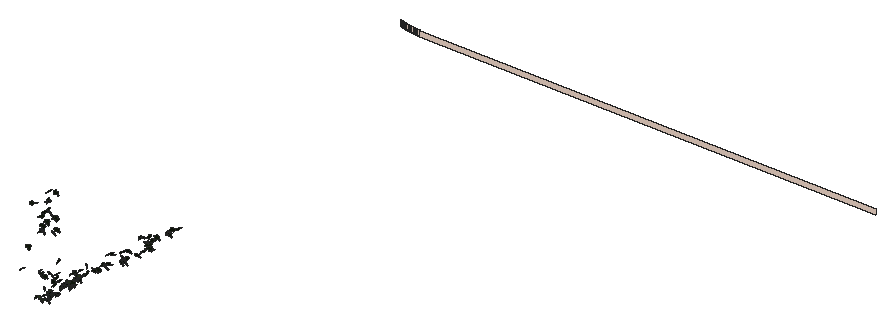
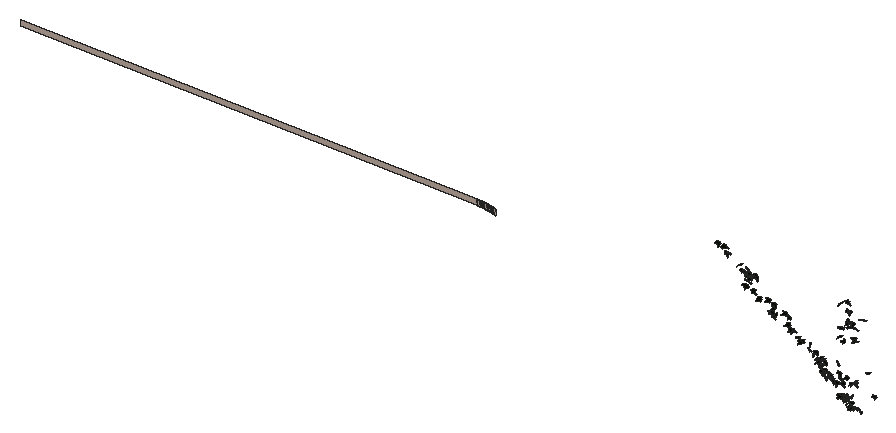
# SketchUp Ruby script. Lengths in inches.
U = 1.inch
M = Sketchup.active_model
def pt(a) = Geom::Point3d.new(a.map { |v| v * U })
def face(e, loops, mat)
  f = e.add_face(loops[0].map { |a| pt(a) })
  loops[1..].each { |l| e.add_face(l.map { |a| pt(a) }).erase! }
  f.material = f.back_material = mat if mat
  f
end
# faces: each face lists its corners as indices into pts; further lists are holes
def faces(e, pts, list, mat = nil) = list.each { |f| face(e, (f[0].is_a?(Array) ? f : [f]).map { |l| l.map { |i| pts[i] } }, mat) }
# xy, xz, yz: faces in a plane at the given z, y or x. An outline is a flat list of corners, or four numbers for a rectangle; further outlines are holes
def ring(l) = l.size == 4 ? [[l[0], l[1]], [l[2], l[1]], [l[2], l[3]], [l[0], l[3]]] : l.each_slice(2).to_a
def flat(e, list, mat, &to3) = list.each { |f| face(e, (f[0].is_a?(Array) ? f : [f]).map { |l| ring(l).map { |u, v| to3.(u, v) } }, mat) }
def xy(e, z, list, mat = nil) = flat(e, list, mat) { |x, y| [x, y, z] }
def xz(e, y, list, mat = nil) = flat(e, list, mat) { |x, z| [x, y, z] }
def yz(e, x, list, mat = nil) = flat(e, list, mat) { |y, z| [x, y, z] }
def lines(e, pts, list) = list.each { |a, b| e.add_line(pt(pts[a]), pt(pts[b])) }
# prism: a flat outline (further loops are holes) pulled along v
def prism(e, loops, v, mat = nil)
  f = face(e, loops, mat); d = Geom::Vector3d.new(v.map { |x| x * U })
  f.pushpull(f.normal.samedirection?(d) ? d.length : -d.length)
end
def box(e, o, s, mat = nil) = prism(e, [[o, [o[0] + s[0], o[1], o[2]], [o[0] + s[0], o[1] + s[1], o[2]], [o[0], o[1] + s[1], o[2]]]], [0, 0, s[2]], mat)
def at(x, y, z, deg = 0) = Geom::Transformation.translation(pt([x, y, z])) * Geom::Transformation.rotation(ORIGIN, Z_AXIS, deg.degrees)
def axes(o, x, y, z) = Geom::Transformation.new([*x, 0, *y, 0, *z, 0, *pt(o).to_a, 1])
def part(name) = M.definitions.add(name)
# library, detail: a bought-in or finely detailed component or shape, given as its bounding box
def library(name, o, s) = part(name).tap { |d| box(d.entities, o, s) }
def detail(e, o, s) = box(e.add_group.entities, o, s)
def put(e, d, t, mat = nil) = e.add_instance(d, t).tap { |i| i.material = mat if mat }
def group(e, t, mat = nil) = e.add_group.tap { |g| g.transformation = t; g.material = mat if mat }.entities
root = M.entities
M.materials.add("1026 AP 7946 SUNNY SIDE UP").color = [254, 231, 186]
M.materials.add("1937 AP K247 Camellia Bud-N").color = [246, 221, 207]
M.materials.add("efeu1").color = [18, 25, 13]
M.materials.add("efeu2").color = [43, 57, 29]
c1 = part("ivyleaf_10")
p = [[0,0.5,-0.03],[-0.0625,2.02,-0.43],[-0.19,2.01,-0.46],[-0.54,1.05,-0.29],[-0.52,0.625,-0.18],[-0.83,0.76,-0.28],
  [-1.16,0.64,-0.33],[-1.15,0.33,-0.24],[-0.77,-0.39,0.02],[-0.3,-0.51,0.16],[0.04,-0.48,0.23],[-0.02,2.01,-0.4375],
  [-0.06,2.01,-0.43],[0.04,-0.49,0.23],[0.67,-0.49,0.14],[1.38,0.36,-0.2],[1.375,0.51,-0.24],[0.81,0.65,-0.19],
  [0.62,0.59,-0.15],[0.6,1.09,-0.28],[0.5,1.23,-0.31]]
faces(c1.entities,p,[[0,1,2,3,4,5,6,7,8,9,10],[11,12,0,13,14,15,16,17,18,19,20]],"efeu2")
c2 = part("ivyleaf_9")
p = [[1.54,2.16,1.25],[1.36,2.04,1.19],[-0.21,0.99,0.68],[-0.71,1.11,0.82],[-0.85,0.86,0.67],[-0.8,0.17,0.21],
  [-0.9,-0.01,0.1],[-0.67,-0.16,-0.02],[-0.08,-0.08,-0.05],[-0.03,-0.6,-0.4],[0.65,-0.88,-0.66],[0.83,-0.6,-0.49],
  [1.29,-0.42,-0.43],[1.8125,-0.07,-0.26],[1.21,0.44,0.15]]
faces(c2.entities,p,[[0,1,2,3,4,5,6,7,8,9,10,11,12,13,14]],"efeu1")
xz(root,299,[[224.73,370,225,372],[225,370,396,372]],"1937 AP K247 Camellia Bud-N")
xz(root,299.01,[[224.2,370,224.47,372]],"1937 AP K247 Camellia Bud-N")
p = [[223.41,299.05,372],[223.15,299.0625,372],[223.15,299.0625,370],[223.41,299.05,370],[223.68,299.03,372],[223.68,299.03,370],
  [223.94,299.02,372],[223.94,299.02,370],[224.2,299.01,372],[224.2,299.01,370],[224.73,299,372],[224.47,299.01,372],
  [224.47,299.01,370],[224.73,299,370],[222.35,299.13,372],[222.09,299.16,372],[222.09,299.16,370],[222.35,299.13,370],
  [222.62,299.11,372],[222.62,299.11,370],[222.88,299.08,372],[222.88,299.08,370],[221.5625,299.22,372],[221.3,299.25,372],
  [221.3,299.25,370],[221.5625,299.22,370],[221.83,299.1875,372],[221.83,299.1875,370],[220.78,299.33,372],[220.51,299.375,372],
  [220.51,299.375,370],[220.78,299.33,370],[221.04,299.29,372],[221.04,299.29,370],[220.25,299.42,372],[219.99,299.47,372],
  [219.99,299.47,370],[220.25,299.42,370],[219.73,299.52,372],[219.47,299.57,372],[219.47,299.57,370],[219.73,299.52,370],
  [219.21,299.63,372],[218.96,299.69,372],[218.96,299.69,370],[219.21,299.63,370],[218.7,299.75,372],[218.44,299.81,372],
  [218.44,299.81,370],[218.7,299.75,370],[218.18,299.875,372],[218.18,299.875,370],[217.93,299.94,372],[217.67,300.01,372],
  [217.67,300.01,370],[217.93,299.94,370],[217.42,300.09,372],[217.42,300.09,370],[217.16,300.16,372],[217.16,300.16,370],
  [216.91,300.24,372],[216.66,300.32,372],[216.66,300.32,370],[216.91,300.24,370]]
faces(root,p,[[0,1,2,3],[4,0,3,5],[6,4,5,7],[8,6,7,9],[10,11,12,13],[14,15,16,17],[18,14,17,19],[20,18,19,21],
  [1,20,21,2],[22,23,24,25],[26,22,25,27],[15,26,27,16],[28,29,30,31],[32,28,31,33],[23,32,33,24],[34,35,36,37],
  [29,34,37,30],[38,39,40,41],[35,38,41,36],[42,43,44,45],[39,42,45,40],[46,47,48,49],[43,46,49,44],[47,50,51,48],
  [52,53,54,55],[50,52,55,51],[53,56,57,54],[56,58,59,57],[60,61,62,63],[58,60,63,59]],"1937 AP K247 Camellia Bud-N")
put(root,c1,axes([149.72,216,291.52],[-0.17011,-0.34982,0.04616],[0.18059,-0.08117,-0.35208],[0.52475,-0.08547,0.13613]),"1026 AP 7946 SUNNY SIDE UP")
put(root,c1,axes([149.96,215.9375,291.71],[-0.41211,-0.26062,-0.0123],[0.05123,-0.01799,-0.3791],[0.40692,-0.26168,0.03527]),"1026 AP 7946 SUNNY SIDE UP")
put(root,c2,axes([151.71,216.18,294.14],[0.05702,-0.34851,0.10563],[0.03455,-0.10275,-0.3614],[0.57107,0.04101,0.01132]),"1026 AP 7946 SUNNY SIDE UP")
put(root,c2,axes([152.55,216.18,293.81],[-0.00015,-0.37303,0.06039],[-0.00756,-0.06073,-0.38462],[0.59423,-0.00087,-0.00488]),"1026 AP 7946 SUNNY SIDE UP")
put(root,c2,axes([154.37,216,298.25],[-0.44324,0.24159,-0.06762],[0.04755,-0.06733,-0.38152],[-0.39134,-0.28181,0.03024]),"1026 AP 7946 SUNNY SIDE UP")
put(root,c1,axes([151.59,216.05,294.53],[0.13663,0.35643,-0.09871],[-0.04004,-0.09449,-0.37849],[-0.5798,0.09052,0.00288]),"1026 AP 7946 SUNNY SIDE UP")
put(root,c2,axes([149.6,216.22,314.85],[-0.67915,0.0452,-0.05361],[0.05432,-0.14548,-0.42433],[-0.09414,-0.41003,0.14191]),"1026 AP 7946 SUNNY SIDE UP")
put(root,c1,axes([148.62,216.08,292.08],[0.52629,-0.11382,-0.05801],[-0.09588,-0.0069,-0.36327],[0.17463,0.33923,-0.02464]),"1026 AP 7946 SUNNY SIDE UP")
put(root,c1,axes([151.9375,215.91,294.43],[0.09275,-0.28891,-0.24916],[-0.05487,0.2379,-0.30219],[0.58825,0.06774,0.0111]),"1026 AP 7946 SUNNY SIDE UP")
put(root,c2,axes([152.52,216.21,294.85],[-0.25319,0.21542,-0.25808],[0.11291,-0.25055,-0.26966],[-0.5086,-0.16286,0.06861]),"1026 AP 7946 SUNNY SIDE UP")
put(root,c2,axes([149.81,216.04,299.81],[0.26931,-0.27079,-0.2448],[-0.10884,0.23177,-0.32424],[0.55431,0.17707,0.05527]),"1026 AP 7946 SUNNY SIDE UP")
put(root,c1,axes([148.83,216.29,301.01],[-0.07493,-0.34442,0.19327],[-0.0523,-0.18674,-0.35923],[0.61597,-0.05775,-0.00699]),"1026 AP 7946 SUNNY SIDE UP")
put(root,c1,axes([150.3125,216,295.59],[-0.24963,0.31574,0.11789],[-0.09076,0.09703,-0.36343],[-0.51925,-0.16875,0.00685]),"1026 AP 7946 SUNNY SIDE UP")
put(root,c2,axes([151.2,216.28,318.45],[-0.18343,-0.39792,-0.18257],[0.18595,0.14527,-0.42074],[0.65772,-0.15205,0.06803]),"1026 AP 7946 SUNNY SIDE UP")
put(root,c2,axes([150.63,215.99,299.73],[0.13417,-0.17103,-0.36413],[-0.08066,0.35277,-0.18706],[0.61075,0.08416,0.05529]),"1026 AP 7946 SUNNY SIDE UP")
put(root,c2,axes([149.15,216.26,314.56],[0.47126,-0.31653,0.00167],[-0.0294,-0.0224,-0.44821],[0.49688,0.29889,-0.0281]),"1026 AP 7946 SUNNY SIDE UP")
put(root,c2,axes([158.375,216.1,299.91],[0.52416,0.13091,-0.17564],[-0.21898,-0.10988,-0.36649],[-0.25868,0.35829,-0.04565]),"1026 AP 7946 SUNNY SIDE UP")
put(root,c2,axes([157.85,216.39,299.3],[-0.56526,-0.10682,-0.08152],[0.13503,-0.01473,-0.38447],[0.15882,-0.36767,0.03675]),"1026 AP 7946 SUNNY SIDE UP")
put(root,c2,axes([151.17,216.38,291.91],[0.30277,-0.30922,0.07791],[0.04857,-0.07187,-0.3755],[0.49885,0.19467,-0.01073]),"1026 AP 7946 SUNNY SIDE UP")
put(root,c2,axes([160.84,216.45,301.19],[-0.56238,-0.15305,0.00027],[0.01955,-0.0319,-0.39941],[0.23987,-0.35623,0.03317]),"1026 AP 7946 SUNNY SIDE UP")
put(root,c2,axes([147.28,216,291.45],[0.05899,0.22927,0.27643],[-0.09594,0.26871,-0.22728],[-0.54503,-0.02249,0.06993]),"1026 AP 7946 SUNNY SIDE UP")
put(root,c2,axes([145.36,216.04,322.64],[0.65967,-0.15991,-0.13381],[0.20046,0.43261,-0.12282],[0.25332,0.07408,0.44565]),"1026 AP 7946 SUNNY SIDE UP")
put(root,c2,axes([149.45,216.11,300.07],[-0.27677,0.30741,0.18647],[-0.18521,0.13839,-0.36283],[-0.52802,-0.20968,0.02953]),"1026 AP 7946 SUNNY SIDE UP")
put(root,c2,axes([150.54,216.14,293.44],[0.12426,0.34712,-0.07049],[-0.04558,-0.06555,-0.36687],[-0.55505,0.08309,0.01435]),"1026 AP 7946 SUNNY SIDE UP")
put(root,c2,axes([161.58,216.59,304.66],[-0.02519,-0.07286,-0.40886],[0.02922,-0.39649,0.07197],[-0.63316,-0.0154,0.01959]),"1026 AP 7946 SUNNY SIDE UP")
put(root,c2,axes([156.92,216.22,298.43],[0.48185,0.18604,-0.1307],[-0.14582,-0.09293,-0.36861],[-0.32369,0.3188,-0.02851]),"1026 AP 7946 SUNNY SIDE UP")
put(root,c1,axes([155.96,216.34,297.66],[-0.24146,0.33983,-0.06349],[0.01896,-0.06424,-0.38423],[-0.54329,-0.15328,0.01481]),"1026 AP 7946 SUNNY SIDE UP")
put(root,c2,axes([151.83,216.39,301.24],[0.5563,-0.17456,0.11322],[0.12394,-0.08933,-0.40447],[0.30064,0.35984,-0.04275]),"1026 AP 7946 SUNNY SIDE UP")
put(root,c2,axes([149.31,216.39,314.9],[0.44466,-0.30642,-0.13757],[-0.16022,0.08517,-0.42873],[0.49942,0.30015,-0.01506]),"1026 AP 7946 SUNNY SIDE UP")
put(root,c2,axes([162.43,216.65,303.75],[-0.59992,-0.09624,-0.03499],[0.09509,-0.10968,-0.38646],[0.12892,-0.36695,0.1222]),"1026 AP 7946 SUNNY SIDE UP")
put(root,c2,axes([170.35,216.75,308.71],[-0.35447,-0.35818,0.08055],[0.04249,-0.11008,-0.42876],[0.57559,-0.21246,0.08126]),"1026 AP 7946 SUNNY SIDE UP")
put(root,c1,axes([152.22,216.37,295.1],[-0.24706,-0.12632,0.31631],[0.34102,0.21919,0.20803],[-0.39666,0.26713,-0.01816]),"1026 AP 7946 SUNNY SIDE UP")
put(root,c2,axes([160.28,216.38,303.7],[-0.17467,0.37956,0.00047],[-0.00785,-0.00323,-0.4074],[-0.59678,-0.11105,0.00522]),"1026 AP 7946 SUNNY SIDE UP")
put(root,c2,axes([154.8,216.32,300.44],[-0.25114,0.4049,0.12691],[-0.1082,0.10259,-0.44704],[-0.65557,-0.17204,0.02516]),"1026 AP 7946 SUNNY SIDE UP")
put(root,c1,axes([157.77,216.48,299.5],[-0.06316,0.38089,-0.00176],[-0.00654,-0.00434,-0.39456],[-0.59891,-0.04012,0.0045]),"1026 AP 7946 SUNNY SIDE UP")
put(root,c2,axes([153.32,216.375,298.76],[0.22721,0.04433,0.39953],[0.61087,0.02102,-0.15157],[-0.05547,0.41309,-0.03271]),"1026 AP 7946 SUNNY SIDE UP")
put(root,c1,axes([161.27,216.51,304.64],[-0.21026,0.37622,-0.03857],[0.00182,-0.04157,-0.41137],[-0.59483,-0.13311,0.01238]),"1026 AP 7946 SUNNY SIDE UP")
put(root,c1,axes([163.14,216.64,303.96],[0.2893,0.30713,-0.17555],[-0.11001,-0.15847,-0.36923],[-0.54258,0.19589,-0.01874]),"1026 AP 7946 SUNNY SIDE UP")
put(root,c2,axes([155.01,216.33,301.98],[-0.03033,0.44677,0.03323],[-0.00488,0.02961,-0.46052],[-0.70405,-0.01945,0.00176]),"1026 AP 7946 SUNNY SIDE UP")
put(root,c1,axes([158.74,216.58,300.76],[-0.60532,-0.02173,-0.0108],[0.02271,-0.07568,-0.3898],[0.03029,-0.3776,0.07644]),"1026 AP 7946 SUNNY SIDE UP")
put(root,c1,axes([151.99,216.37,294.98],[-0.01393,-0.22348,-0.30159],[0.08359,0.28772,-0.22723],[0.57146,-0.04753,0.02589]),"1026 AP 7946 SUNNY SIDE UP")
put(root,c1,axes([164.32,216.89,304.61],[-0.04953,0.03206,-0.40968],[-0.01707,-0.39902,-0.03457],[-0.62739,0.00833,0.03328]),"1026 AP 7946 SUNNY SIDE UP")
put(root,c2,axes([168.9375,216.61,307.51],[0.30285,-0.06673,0.38541],[-0.49335,0.20946,0.20591],[-0.33817,-0.36533,0.04475]),"1026 AP 7946 SUNNY SIDE UP")
put(root,c2,axes([162.13,216.48,302.61],[0.50656,-0.07707,-0.24925],[-0.36325,0.07156,-0.34057],[0.16414,0.39622,0.01551]),"1026 AP 7946 SUNNY SIDE UP")
put(root,c2,axes([153.84,216.53,294.88],[0.54344,-0.01201,-0.16946],[-0.25923,-0.02723,-0.3551],[-0.00139,0.38176,-0.02841]),"1026 AP 7946 SUNNY SIDE UP")
put(root,c2,axes([162.61,216.71,303.36],[-0.14323,0.25551,-0.29512],[-0.00769,-0.29662,-0.27131],[-0.60524,-0.0567,0.07329]),"1026 AP 7946 SUNNY SIDE UP")
put(root,c2,axes([163.64,216.55,306.14],[-0.01877,0.37701,-0.16117],[-0.01934,-0.15891,-0.38917],[-0.64283,-0.00622,0.01642]),"1026 AP 7946 SUNNY SIDE UP")
put(root,c2,axes([166.08,216.8125,306.25],[-0.45917,0.10898,-0.29049],[0.33764,-0.20235,-0.31016],[-0.33587,-0.3524,0.08533]),"1026 AP 7946 SUNNY SIDE UP")
put(root,c2,axes([161.11,216.46,300.41],[0.2563,0.35263,-0.10001],[-0.1416,-0.06654,-0.39698],[-0.55827,0.17877,0.05478]),"1026 AP 7946 SUNNY SIDE UP")
put(root,c2,axes([149.38,216.77,319.3],[-0.59701,0.24301,-0.0114],[-0.09507,-0.11656,-0.44512],[-0.3706,-0.36156,0.13255]),"1026 AP 7946 SUNNY SIDE UP")
put(root,c2,axes([162.875,216.75,302.92],[0.25699,-0.34645,-0.10329],[-0.07264,0.08688,-0.3941],[0.56159,0.16978,-0.00371]),"1026 AP 7946 SUNNY SIDE UP")
put(root,c1,axes([152.95,216.86,294.125],[-0.09025,-0.34029,0.15929],[-0.00178,-0.15823,-0.35565],[0.58898,-0.05262,0.02333]),"1026 AP 7946 SUNNY SIDE UP")
put(root,c1,axes([159.22,216.86,298.99],[0.00748,0.31414,-0.24843],[-0.04466,-0.24206,-0.32445],[-0.62283,0.02113,0.02028]),"1026 AP 7946 SUNNY SIDE UP")
put(root,c2,axes([150.26,216.71,291.77],[0.53029,-0.14782,0.03668],[0.02989,-0.04701,-0.37787],[0.23751,0.33594,-0.03435]),"1026 AP 7946 SUNNY SIDE UP")
put(root,c2,axes([151.47,216.84,293.02],[0.2014,-0.34908,-0.04538],[-0.03251,0.03722,-0.38279],[0.55191,0.12957,-0.00599]),"1026 AP 7946 SUNNY SIDE UP")
put(root,c1,axes([159.81,216.82,298.52],[0.35324,-0.32642,-0.0169],[-0.04934,-0.00397,-0.40721],[0.51139,0.22509,-0.02761]),"1026 AP 7946 SUNNY SIDE UP")
put(root,c2,axes([149.18,217.01,315.89],[-0.34447,-0.3602,-0.13737],[0.21212,0.06913,-0.42684],[0.56428,-0.24587,0.0766]),"1026 AP 7946 SUNNY SIDE UP")
put(root,c1,axes([162.68,216.78,303.86],[0.28303,0.34853,0.05898],[0.04346,0.04794,-0.40382],[-0.55318,0.18209,-0.00155]),"1026 AP 7946 SUNNY SIDE UP")
put(root,c1,axes([160.54,216.88,300.06],[-0.58502,0.01714,-0.15398],[0.23036,-0.05057,-0.38171],[-0.0545,-0.39779,0.03952]),"1026 AP 7946 SUNNY SIDE UP")
put(root,c2,axes([141.55,216.71,298.88],[0.05723,0.37892,0.03321],[-0.01635,0.0312,-0.39174],[-0.59747,0.03544,0.0139]),"1026 AP 7946 SUNNY SIDE UP")
put(root,c1,axes([161.28,216.85,302.46],[-0.28725,-0.31148,-0.16038],[0.20331,0.10045,-0.36693],[0.50706,-0.21673,0.05627]),"1026 AP 7946 SUNNY SIDE UP")
put(root,c2,axes([171.67,217.05,310.78],[-0.50806,0.19674,-0.18361],[0.17228,-0.15877,-0.38371],[-0.38151,-0.3337,0.07124]),"1026 AP 7946 SUNNY SIDE UP")
put(root,c2,axes([165.53,216.8125,308.12],[0.2702,-0.06743,-0.38206],[-0.5158,0.17318,-0.18821],[0.29077,0.36986,0.02118]),"1026 AP 7946 SUNNY SIDE UP")
put(root,c2,axes([178.88,216.99,315.7],[0.64597,-0.14467,-0.0357],[-0.07474,-0.03372,-0.44622],[0.22134,0.41082,-0.04648]),"1026 AP 7946 SUNNY SIDE UP")
put(root,c2,axes([173.4,216.84,311.72],[0.53542,0.09778,0.26367],[0.39718,0.04384,-0.36398],[-0.16478,0.42338,-0.02057]),"1026 AP 7946 SUNNY SIDE UP")
put(root,c1,axes([152.28,216.99,293.76],[0.53294,0.07942,0.14979],[0.18495,0.11643,-0.34837],[-0.18258,0.34975,0.08434]),"1026 AP 7946 SUNNY SIDE UP")
put(root,c2,axes([153.44,216.96,294.625],[0.53326,-0.16128,-0.06203],[-0.00391,0.12658,-0.36857],[0.27016,0.32017,0.11711]),"1026 AP 7946 SUNNY SIDE UP")
put(root,c2,axes([149.74,216.92,320.73],[0.16348,0.43976,-0.05759],[0.00886,-0.06129,-0.46546],[-0.6975,0.10229,-0.01941]),"1026 AP 7946 SUNNY SIDE UP")
put(root,c2,axes([171.93,217.16,310.18],[0.54684,-0.19994,0.12265],[0.14797,-0.07718,-0.41324],[0.33565,0.35977,-0.01764]),"1026 AP 7946 SUNNY SIDE UP")
put(root,c2,axes([168.91,217.08,307.84],[0.63347,0.02555,-0.07442],[-0.11355,-0.00498,-0.41589],[-0.04092,0.40929,0.00199]),"1026 AP 7946 SUNNY SIDE UP")
put(root,c2,axes([174.51,217,315.23],[0.50441,0.13346,0.26335],[0.37135,0.09587,-0.35737],[-0.25836,0.39834,0.0005]),"1026 AP 7946 SUNNY SIDE UP")
put(root,c2,axes([177.9375,217.29,313.6875],[0.47233,-0.31696,-0.09194],[-0.11962,0.04822,-0.44904],[0.50298,0.30912,-0.02046]),"1026 AP 7946 SUNNY SIDE UP")
put(root,c2,axes([179.19,217.29,314.11],[0.63908,-0.17744,0.05334],[0.04996,-0.05859,-0.45528],[0.28678,0.40564,-0.03955]),"1026 AP 7946 SUNNY SIDE UP")
put(root,c2,axes([154.17,217.08,294.81],[0.50756,0.18819,0.07813],[0.09266,0.04733,-0.38448],[-0.30463,0.32795,0.01324]),"1026 AP 7946 SUNNY SIDE UP")
put(root,c2,axes([150.79,217.13,324.45],[0.14207,0.44367,-0.11435],[-0.11309,-0.10052,-0.46431],[-0.71117,0.10462,0.05099]),"1026 AP 7946 SUNNY SIDE UP")
put(root,c2,axes([150.98,217.48,324.89],[-0.59178,0.08051,-0.27389],[0.38558,-0.11567,-0.3937],[-0.20669,-0.44631,0.04976]),"1026 AP 7946 SUNNY SIDE UP")
put(root,c2,axes([173.22,216.97,314.42],[0.23876,0.33104,0.2348],[0.01415,0.23884,-0.36517],[-0.63014,0.13079,0.08076]),"1026 AP 7946 SUNNY SIDE UP")
put(root,c2,axes([154.78,217.47,305.9],[-0.4742,0.1688,-0.27641],[0.33792,-0.16514,-0.35558],[-0.36813,-0.36902,0.02965]),"1026 AP 7946 SUNNY SIDE UP")
put(root,c2,axes([188.03,217,324.16],[0.15983,0.31845,0.34355],[0.13583,0.3204,-0.34232],[-0.71012,0.13296,0.01185]),"1026 AP 7946 SUNNY SIDE UP")
put(root,c2,axes([160.34,217.53,299.83],[-0.61503,0.0738,0.02499],[-0.04638,-0.02822,-0.4088],[-0.11279,-0.39085,0.03186]),"1026 AP 7946 SUNNY SIDE UP")
put(root,c2,axes([178.6,217.32,317.1875],[0.00005,0.42052,-0.11512],[-0.00486,-0.11414,-0.43387],[-0.68513,0.00084,0.00307]),"1026 AP 7946 SUNNY SIDE UP")
put(root,c2,axes([154.91,217.26,299.22],[0.19014,0.42292,0.06809],[0.04659,0.05775,-0.45263],[-0.67088,0.12387,-0.01213]),"1026 AP 7946 SUNNY SIDE UP")
put(root,c2,axes([150.79,217.58,321.61],[-0.50791,0.29793,-0.13062],[0.06704,-0.14075,-0.44748],[-0.50575,-0.31786,0.07186]),"1026 AP 7946 SUNNY SIDE UP")
put(root,c2,axes([142.93,217.69,306.66],[-0.16067,-0.3795,-0.128],[0.2011,0.08818,-0.39209],[0.59371,-0.13257,0.09817]),"1026 AP 7946 SUNNY SIDE UP")
put(root,c2,axes([172.38,217.32,310.83],[0.11679,0.41063,0.04217],[0.04092,0.03448,-0.42923],[-0.64723,0.07628,-0.01953]),"1026 AP 7946 SUNNY SIDE UP")
put(root,c2,axes([188.58,217.83,323.17],[-0.70183,-0.05534,0.08503],[-0.11681,-0.06858,-0.45988],[0.1044,-0.44875,0.05707]),"1026 AP 7946 SUNNY SIDE UP")
put(root,c2,axes([185.4,217.55,324.0625],[-0.13612,0.45213,-0.05026],[0.00207,-0.05202,-0.47447],[-0.7155,-0.08616,0.00819]),"1026 AP 7946 SUNNY SIDE UP")
put(root,c2,axes([151.0625,217.64,327.86],[-0.30275,0.42506,-0.10099],[-0.06058,-0.12587,-0.4734],[-0.6841,-0.17697,0.08661]),"1026 AP 7946 SUNNY SIDE UP")
put(root,c2,axes([188.73,217.73,325.84],[-0.56361,0.28516,-0.04259],[0.01776,-0.05459,-0.47076],[-0.4531,-0.35685,0.03452]),"1026 AP 7946 SUNNY SIDE UP")
put(root,c2,axes([188.85,217.76,321.8125],[-0.60221,0.23976,0.13236],[-0.23994,-0.00845,-0.45726],[-0.35286,-0.40344,0.08504]),"1026 AP 7946 SUNNY SIDE UP")
put(root,c2,axes([180.36,217.63,318.11],[0.70595,0.07454,0.04771],[0.08455,-0.04564,-0.46586],[-0.10861,0.44899,-0.05255]),"1026 AP 7946 SUNNY SIDE UP")
put(root,c2,axes([150.51,217.76,320.79],[0.66884,-0.15676,-0.033],[-0.06293,-0.01874,-0.46601],[0.24331,0.42609,-0.0298]),"1026 AP 7946 SUNNY SIDE UP")
put(root,c2,axes([151.88,218.05,314.11],[0.40327,-0.28889,0.22103],[0.17604,-0.18843,-0.39733],[0.53936,0.2775,-0.03557]),"1026 AP 7946 SUNNY SIDE UP")
put(root,c2,axes([189.41,218.07,324.68],[-0.63517,0.10136,-0.19923],[0.23638,-0.1674,-0.41364],[-0.25009,-0.41566,0.11503]),"1026 AP 7946 SUNNY SIDE UP")
put(root,c2,axes([185.13,217.63,324.3125],[0.55152,0.24186,0.18027],[0.24605,0.07847,-0.43785],[-0.39826,0.38342,-0.02088]),"1026 AP 7946 SUNNY SIDE UP")
put(root,c2,axes([186.88,217.86,323.15],[0.7144,-0.01363,0.00193],[0.00101,-0.04354,-0.46637],[0.02163,0.45225,-0.04217]),"1026 AP 7946 SUNNY SIDE UP")
put(root,c2,axes([190.36,218.02,324.79],[-0.39853,0.33613,-0.19371],[0.10029,-0.18764,-0.43086],[-0.59875,-0.25516,0.05677]),"1026 AP 7946 SUNNY SIDE UP")
put(root,c2,axes([190.8,218.09,326.38],[0.11948,-0.40636,-0.21778],[0.04513,0.21579,-0.42003],[0.71717,0.05412,0.06272]),"1026 AP 7946 SUNNY SIDE UP")
put(root,c2,axes([196.92,218.35,330.8],[-0.12459,0.11192,-0.46975],[-0.12509,-0.45957,-0.10451],[-0.72858,0.05977,0.09827]),"1026 AP 7946 SUNNY SIDE UP")
put(root,c2,axes([195.2,218.25,328.96],[-0.22056,-0.27677,-0.36943],[0.47181,0.22238,-0.29774],[0.53099,-0.31256,0.11111]),"1026 AP 7946 SUNNY SIDE UP")
put(root,c2,axes([183.12,218.09,317.56],[0.6844,-0.01196,0.14754],[0.22396,-0.02657,-0.44818],[0.03089,0.45746,-0.01949]),"1026 AP 7946 SUNNY SIDE UP")
put(root,c2,axes([185.82,218.25,319.62],[-0.1367,0.36761,-0.27568],[-0.00916,-0.27542,-0.38643],[-0.71684,-0.06658,0.05751]),"1026 AP 7946 SUNNY SIDE UP")
put(root,c2,axes([153.14,218.17,315.66],[0.09438,-0.33047,-0.31567],[0.00178,0.30736,-0.34157],[0.70664,0.04336,0.04303]),"1026 AP 7946 SUNNY SIDE UP")
put(root,c2,axes([153.17,218.65,318.88],[-0.5439,-0.09472,0.29532],[-0.38873,-0.16275,-0.36299],[0.27388,-0.4191,0.07127]),"1026 AP 7946 SUNNY SIDE UP")
put(root,c2,axes([179.53,218.625,314.77],[-0.61559,0.21548,0.02607],[-0.07802,-0.04064,-0.45652],[-0.33188,-0.39013,0.05895]),"1026 AP 7946 SUNNY SIDE UP")
put(root,c2,axes([178.11,218.42,313.8],[-0.15633,0.41672,0.125],[-0.19273,0.09004,-0.4299],[-0.65361,-0.12622,0.09687]),"1026 AP 7946 SUNNY SIDE UP")
put(root,c2,axes([195.47,218.41,329.03],[-0.00327,0.47137,0.02011],[-0.04384,0.01669,-0.48467],[-0.74036,-0.00307,0.02861]),"1026 AP 7946 SUNNY SIDE UP")
put(root,c2,axes([152.23,218.78,319.15],[-0.33115,-0.219,-0.35293],[0.48843,0.16017,-0.30237],[0.40998,-0.36771,0.07516]),"1026 AP 7946 SUNNY SIDE UP")
put(root,c2,axes([198.5625,218.59,331.53],[0.17562,0.46515,-0.00194],[0.01758,-0.00734,-0.49268],[-0.73122,0.11154,-0.01231]),"1026 AP 7946 SUNNY SIDE UP")
put(root,c2,axes([187.94,218.8,320.81],[0.59762,0.2474,-0.11155],[-0.12877,-0.0751,-0.46727],[-0.40559,0.38839,-0.01601]),"1026 AP 7946 SUNNY SIDE UP")
put(root,c2,axes([152.16,219.05,327.47],[0.19397,-0.40537,-0.22552],[-0.06429,0.2137,-0.43476],[0.71983,0.12832,0.02194]),"1026 AP 7946 SUNNY SIDE UP")
